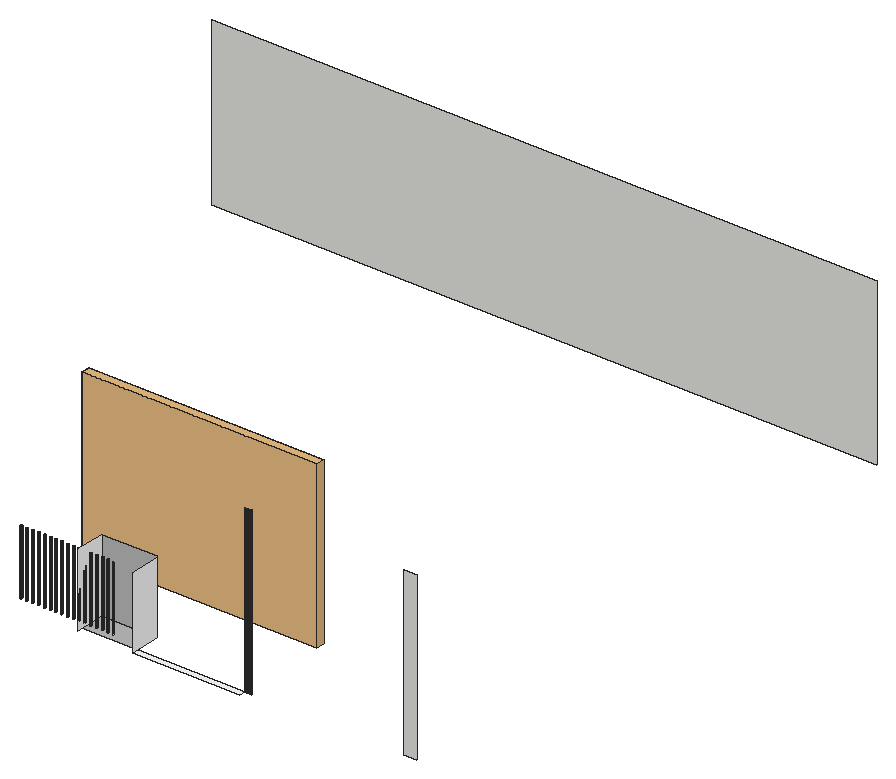
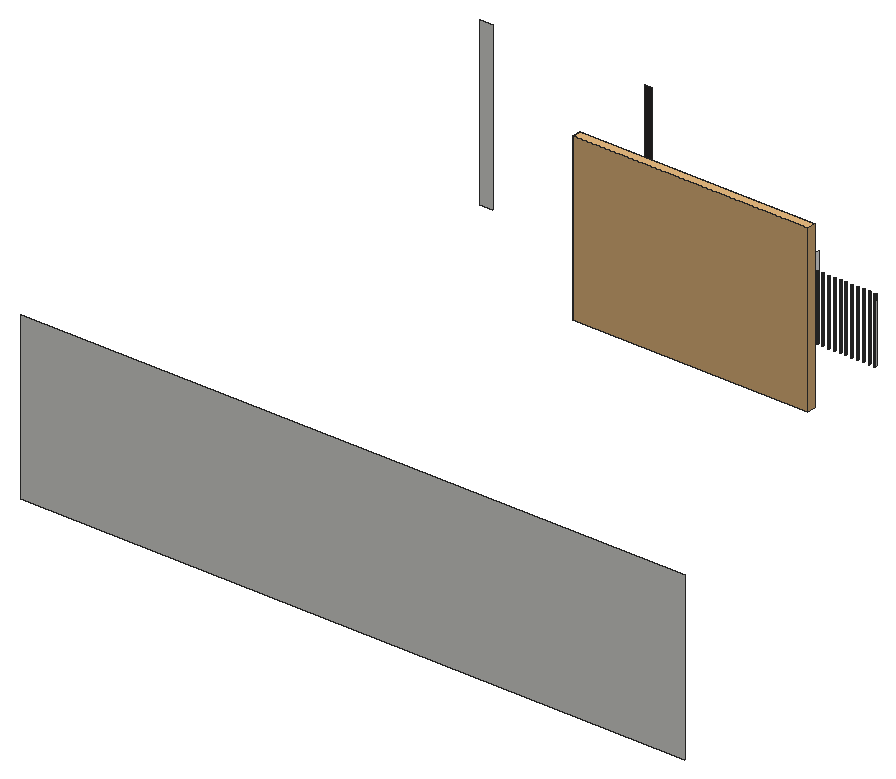
# SketchUp Ruby script. Lengths in inches.
U = 1.inch
M = Sketchup.active_model
def pt(a) = Geom::Point3d.new(a.map { |v| v * U })
def face(e, loops, mat)
  f = e.add_face(loops[0].map { |a| pt(a) })
  loops[1..].each { |l| e.add_face(l.map { |a| pt(a) }).erase! }
  f.material = f.back_material = mat if mat
  f
end
# faces: each face lists its corners as indices into pts; further lists are holes
def faces(e, pts, list, mat = nil) = list.each { |f| face(e, (f[0].is_a?(Array) ? f : [f]).map { |l| l.map { |i| pts[i] } }, mat) }
# xy, xz, yz: faces in a plane at the given z, y or x. An outline is a flat list of corners, or four numbers for a rectangle; further outlines are holes
def ring(l) = l.size == 4 ? [[l[0], l[1]], [l[2], l[1]], [l[2], l[3]], [l[0], l[3]]] : l.each_slice(2).to_a
def flat(e, list, mat, &to3) = list.each { |f| face(e, (f[0].is_a?(Array) ? f : [f]).map { |l| ring(l).map { |u, v| to3.(u, v) } }, mat) }
def xy(e, z, list, mat = nil) = flat(e, list, mat) { |x, y| [x, y, z] }
def xz(e, y, list, mat = nil) = flat(e, list, mat) { |x, z| [x, y, z] }
def yz(e, x, list, mat = nil) = flat(e, list, mat) { |y, z| [x, y, z] }
def lines(e, pts, list) = list.each { |a, b| e.add_line(pt(pts[a]), pt(pts[b])) }
# prism: a flat outline (further loops are holes) pulled along v
def prism(e, loops, v, mat = nil)
  f = face(e, loops, mat); d = Geom::Vector3d.new(v.map { |x| x * U })
  f.pushpull(f.normal.samedirection?(d) ? d.length : -d.length)
end
def box(e, o, s, mat = nil) = prism(e, [[o, [o[0] + s[0], o[1], o[2]], [o[0] + s[0], o[1] + s[1], o[2]], [o[0], o[1] + s[1], o[2]]]], [0, 0, s[2]], mat)
def at(x, y, z, deg = 0) = Geom::Transformation.translation(pt([x, y, z])) * Geom::Transformation.rotation(ORIGIN, Z_AXIS, deg.degrees)
def axes(o, x, y, z) = Geom::Transformation.new([*x, 0, *y, 0, *z, 0, *pt(o).to_a, 1])
def part(name) = M.definitions.add(name)
# library, detail: a bought-in or finely detailed component or shape, given as its bounding box
def library(name, o, s) = part(name).tap { |d| box(d.entities, o, s) }
def detail(e, o, s) = box(e.add_group.entities, o, s)
def put(e, d, t, mat = nil) = e.add_instance(d, t).tap { |i| i.material = mat if mat }
def group(e, t, mat = nil) = e.add_group.tap { |g| g.transformation = t; g.material = mat if mat }.entities
root = M.entities
M.materials.add("Generic\#2").color = [186, 186, 186]
M.materials.add("Generic\#4").color = [48, 45, 45]
M.materials.add("[Color M00]").color = [255, 255, 255]
c1 = library("Group\#9",[0,0,0],[238.3125,8.75,168])
xy(root,614.8125,[[294.98,132.01,294.77,132.04,294.58,132.125,294.41,132.25,294.28,132.42,294.2,132.62,294.17,132.83,294.2,133.04,294.28,133.23,294.41,133.4,294.58,133.53,294.77,133.61,294.98,133.64,295.19,133.61,295.39,133.53,295.56,133.4,295.6875,133.23,295.77,133.04,295.8,132.83,295.77,132.62,295.6875,132.42,295.56,132.25,295.39,132.125,295.19,132.04]])
xy(root,614.8125,[[363.4375,124.5,419.5625,149.5]],"Generic\#2")
xy(root,614.8125,[[419.5625,118.5625,528.75,124.5]],"[Color M00]")
xz(root,124.5,[[690.4375,614.8125,703.6875,782.8125]])
xz(root,124.5,[[528.75,614.8125,535.75,782.8125]],"Generic\#4")
xz(root,149.5,[[363.4375,614.8125,419.5625,689.33]],"Generic\#2")
xz(root,724.5,[[15.3125,614.8125,690.4375,782.8125]])
yz(root,363.4375,[[118.5625,614.8125,149.5,689.33]],"[Color M00]")
yz(root,419.5625,[[118.5625,614.8125,149.5,687.77]],"[Color M00]")
p = [[294.58,132.125,614.8125],[294.77,132.04,614.8125],[294.77,132.04,680.58],[294.58,132.125,680.58],[294.98,132.01,614.8125],[294.98,132.01,680.58],
  [295.19,132.04,614.8125],[295.19,132.04,680.58],[295.39,132.125,614.8125],[295.39,132.125,680.58],[300.58,132.125,614.8125],[300.77,132.04,614.8125],
  [300.77,132.04,680.58],[300.58,132.125,680.58],[300.98,132.01,614.8125],[300.98,132.01,680.58],[301.19,132.04,614.8125],[301.19,132.04,680.58],
  [301.39,132.125,614.8125],[301.39,132.125,680.58],[306.51,132.125,614.8125],[306.71,132.04,614.8125],[306.71,132.04,680.58],[306.51,132.125,680.58],
  [306.92,132.01,614.8125],[306.92,132.01,680.58],[307.13,132.04,614.8125],[307.13,132.04,680.58],[307.33,132.125,614.8125],[307.33,132.125,680.58],
  [312.39,132.125,614.8125],[312.58,132.04,614.8125],[312.58,132.04,680.58],[312.39,132.125,680.58],[312.8,132.01,614.8125],[312.8,132.01,680.58],
  [313.01,132.04,614.8125],[313.01,132.04,680.58],[313.2,132.125,614.8125],[313.2,132.125,680.58],[318.33,132.125,614.8125],[318.52,132.04,614.8125],
  [318.52,132.04,680.58],[318.33,132.125,680.58],[318.73,132.01,614.8125],[318.73,132.01,680.58],[318.94,132.04,614.8125],[318.94,132.04,680.58],
  [319.14,132.125,614.8125],[319.14,132.125,680.58],[324.58,132.125,614.8125],[324.77,132.04,614.8125],[324.77,132.04,680.58],[324.58,132.125,680.58],
  [324.98,132.01,614.8125],[324.98,132.01,680.58],[325.19,132.04,614.8125],[325.19,132.04,680.58],[325.39,132.125,614.8125],[325.39,132.125,680.58],
  [330.08,132.125,614.8125],[330.27,132.04,614.8125],[330.27,132.04,680.58],[330.08,132.125,680.58],[330.48,132.01,614.8125],[330.48,132.01,680.58],
  [330.69,132.04,614.8125],[330.69,132.04,680.58],[330.89,132.125,614.8125],[330.89,132.125,680.58],[336.14,132.07,614.8125],[336.36,132.04,614.8125],
  [336.36,132.04,680.58],[336.14,132.07,680.58],[336.57,132.07,614.8125],[336.57,132.07,680.58],[342.02,132.07,614.8125],[342.23,132.04,614.8125],
  [342.23,132.04,680.58],[342.02,132.07,680.58],[342.44,132.07,614.8125],[342.44,132.07,680.58],[348.02,132.07,614.8125],[348.23,132.04,614.8125],
  [348.23,132.04,680.58],[348.02,132.07,680.58],[348.44,132.07,614.8125],[348.44,132.07,680.58],[353.58,132.07,614.8125],[353.79,132.04,614.8125],
  [353.79,132.04,680.58],[353.58,132.07,680.58],[354,132.07,614.8125],[354,132.07,680.58],[359.64,132.07,614.8125],[359.86,132.04,614.8125],
  [359.86,132.04,680.58],[359.64,132.07,680.58],[360.07,132.07,614.8125],[360.07,132.07,680.58],[365.46,132.07,614.8125],[365.67,132.04,614.8125],
  [365.67,132.04,680.58],[365.46,132.07,680.58],[365.88,132.07,614.8125],[365.88,132.07,680.58],[371.27,132.07,614.8125],[371.48,132.04,614.8125],
  [371.48,132.04,680.58],[371.27,132.07,680.58],[371.69,132.07,614.8125],[371.69,132.07,680.58],[377.21,132.07,614.8125],[377.42,132.04,614.8125],
  [377.42,132.04,680.58],[377.21,132.07,680.58],[377.63,132.07,614.8125],[377.63,132.07,680.58],[383.02,132.07,614.8125],[383.23,132.04,614.8125],
  [383.23,132.04,680.58],[383.02,132.07,680.58],[383.44,132.07,614.8125],[383.44,132.07,680.58],[388.96,132.07,614.8125],[389.17,132.04,614.8125],
  [389.17,132.04,680.58],[388.96,132.07,680.58],[294.41,132.25,614.8125],[294.41,132.25,680.58],[295.56,132.25,614.8125],[295.56,132.25,680.58],
  [300.41,132.25,614.8125],[300.41,132.25,680.58],[301.56,132.25,614.8125],[301.56,132.25,680.58],[306.35,132.25,614.8125],[306.35,132.25,680.58],
  [307.49,132.25,614.8125],[307.49,132.25,680.58],[312.22,132.25,614.8125],[312.22,132.25,680.58],[313.37,132.25,614.8125],[313.37,132.25,680.58],
  [318.16,132.25,614.8125],[318.16,132.25,680.58],[319.31,132.25,614.8125],[319.31,132.25,680.58],[324.41,132.25,614.8125],[324.41,132.25,680.58],
  [325.56,132.25,614.8125],[325.56,132.25,680.58],[329.91,132.25,614.8125],[329.91,132.25,680.58],[331.06,132.25,614.8125],[331.06,132.25,680.58],
  [335.95,132.15,614.8125],[335.95,132.15,680.58],[336.76,132.15,614.8125],[336.76,132.15,680.58],[341.82,132.15,614.8125],[341.82,132.15,680.58],
  [342.64,132.15,614.8125],[342.64,132.15,680.58],[347.82,132.15,614.8125],[347.82,132.15,680.58],[348.64,132.15,614.8125],[348.64,132.15,680.58],
  [353.39,132.15,614.8125],[353.39,132.15,680.58],[354.2,132.15,614.8125],[354.2,132.15,680.58],[359.45,132.15,614.8125],[359.45,132.15,680.58],
  [360.26,132.15,614.8125],[360.26,132.15,680.58],[365.26,132.15,614.8125],[365.26,132.15,680.58],[366.07,132.15,614.8125],[366.07,132.15,680.58],
  [371.07,132.15,614.8125],[371.07,132.15,680.58],[371.89,132.15,614.8125],[371.89,132.15,680.58],[377.01,132.15,614.8125],[377.01,132.15,680.58],
  [377.82,132.15,614.8125],[377.82,132.15,680.58],[382.82,132.15,614.8125],[382.82,132.15,680.58],[383.64,132.15,614.8125],[383.64,132.15,680.58],
  [388.76,132.15,614.8125],[388.76,132.15,680.58],[335.78,132.28,614.8125],[335.78,132.28,680.58],[336.93,132.28,614.8125],[336.93,132.28,680.58],
  [341.66,132.28,614.8125],[341.66,132.28,680.58],[342.8,132.28,614.8125],[342.8,132.28,680.58],[347.66,132.28,614.8125],[347.66,132.28,680.58],
  [348.8,132.28,614.8125],[348.8,132.28,680.58],[353.22,132.28,614.8125],[353.22,132.28,680.58],[354.37,132.28,614.8125],[354.37,132.28,680.58],
  [359.28,132.28,614.8125],[359.28,132.28,680.58],[360.43,132.28,614.8125],[360.43,132.28,680.58],[365.09,132.28,614.8125],[365.09,132.28,680.58],
  [366.24,132.28,614.8125],[366.24,132.28,680.58],[370.91,132.28,614.8125],[370.91,132.28,680.58],[372.05,132.28,614.8125],[372.05,132.28,680.58],
  [376.84,132.28,614.8125],[376.84,132.28,680.58],[377.99,132.28,614.8125],[377.99,132.28,680.58],[382.66,132.28,614.8125],[382.66,132.28,680.58],
  [383.8,132.28,614.8125],[383.8,132.28,680.58],[388.59,132.28,614.8125],[388.59,132.28,680.58],[294.28,132.42,614.8125],[294.28,132.42,680.58],
  [295.6875,132.42,614.8125],[295.6875,132.42,680.58],[300.28,132.42,614.8125],[300.28,132.42,680.58],[301.6875,132.42,614.8125],[301.6875,132.42,680.58],
  [306.22,132.42,614.8125],[306.22,132.42,680.58],[307.625,132.42,614.8125],[307.625,132.42,680.58],[312.09,132.42,614.8125],[312.09,132.42,680.58],
  [313.5,132.42,614.8125],[313.5,132.42,680.58],[318.03,132.42,614.8125],[318.03,132.42,680.58],[319.4375,132.42,614.8125],[319.4375,132.42,680.58],
  [324.28,132.42,614.8125],[324.28,132.42,680.58],[325.6875,132.42,614.8125],[325.6875,132.42,680.58],[329.78,132.42,614.8125],[329.78,132.42,680.58],
  [331.1875,132.42,614.8125],[331.1875,132.42,680.58],[335.65,132.45,614.8125],[335.65,132.45,680.58],[337.06,132.45,614.8125],[337.06,132.45,680.58],
  [341.53,132.45,614.8125],[341.53,132.45,680.58],[342.93,132.45,614.8125],[342.93,132.45,680.58],[347.53,132.45,614.8125],[347.53,132.45,680.58],
  [348.93,132.45,614.8125],[348.93,132.45,680.58],[353.09,132.45,614.8125],[353.09,132.45,680.58],[354.5,132.45,614.8125],[354.5,132.45,680.58],
  [359.15,132.45,614.8125],[359.15,132.45,680.58],[360.56,132.45,614.8125],[360.56,132.45,680.58],[364.96,132.45,614.8125],[364.96,132.45,680.58],
  [366.37,132.45,614.8125],[366.37,132.45,680.58],[370.78,132.45,614.8125],[370.78,132.45,680.58],[372.18,132.45,614.8125],[372.18,132.45,680.58],
  [376.71,132.45,614.8125],[376.71,132.45,680.58],[378.12,132.45,614.8125],[378.12,132.45,680.58],[382.53,132.45,614.8125],[382.53,132.45,680.58],
  [383.93,132.45,614.8125],[383.93,132.45,680.58],[388.46,132.45,614.8125],[388.46,132.45,680.58],[294.2,132.62,614.8125],[294.2,132.62,680.58],
  [295.77,132.62,614.8125],[295.77,132.62,680.58],[300.2,132.62,614.8125],[300.2,132.62,680.58],[301.77,132.62,614.8125],[301.77,132.62,680.58],
  [306.14,132.62,614.8125],[306.14,132.62,680.58],[307.7,132.62,614.8125],[307.7,132.62,680.58],[312.01,132.62,614.8125],[312.01,132.62,680.58],
  [313.58,132.62,614.8125],[313.58,132.62,680.58],[317.95,132.62,614.8125],[317.95,132.62,680.58],[319.52,132.62,614.8125],[319.52,132.62,680.58],
  [324.2,132.62,614.8125],[324.2,132.62,680.58],[325.77,132.62,614.8125],[325.77,132.62,680.58],[329.7,132.62,614.8125],[329.7,132.62,680.58],
  [331.27,132.62,614.8125],[331.27,132.62,680.58],[335.57,132.64,614.8125],[335.57,132.64,680.58],[337.14,132.64,614.8125],[337.14,132.64,680.58],
  [341.45,132.64,614.8125],[341.45,132.64,680.58],[343.02,132.64,614.8125],[343.02,132.64,680.58],[347.45,132.64,614.8125],[347.45,132.64,680.58],
  [349.02,132.64,614.8125],[349.02,132.64,680.58],[353.01,132.64,614.8125],[353.01,132.64,680.58],[354.58,132.64,614.8125],[354.58,132.64,680.58],
  [359.07,132.64,614.8125],[359.07,132.64,680.58],[360.64,132.64,614.8125],[360.64,132.64,680.58],[364.88,132.64,614.8125],[364.88,132.64,680.58],
  [366.45,132.64,614.8125],[366.45,132.64,680.58],[370.7,132.64,614.8125],[370.7,132.64,680.58],[372.27,132.64,614.8125],[372.27,132.64,680.58],
  [376.63,132.64,614.8125],[376.63,132.64,680.58],[378.2,132.64,614.8125],[378.2,132.64,680.58],[382.45,132.64,614.8125],[382.45,132.64,680.58],
  [384.02,132.64,614.8125],[384.02,132.64,680.58],[388.38,132.64,614.8125],[388.38,132.64,680.58],[294.17,132.83,614.8125],[294.17,132.83,680.58],
  [295.8,132.83,614.8125],[295.8,132.83,680.58],[300.17,132.83,614.8125],[300.17,132.83,680.58],[301.8,132.83,614.8125],[301.8,132.83,680.58],
  [306.11,132.83,614.8125],[306.11,132.83,680.58],[307.73,132.83,614.8125],[307.73,132.83,680.58],[311.98,132.83,614.8125],[311.98,132.83,680.58],
  [313.61,132.83,614.8125],[313.61,132.83,680.58],[317.92,132.83,614.8125],[317.92,132.83,680.58],[319.55,132.83,614.8125],[319.55,132.83,680.58],
  [324.17,132.83,614.8125],[324.17,132.83,680.58],[325.8,132.83,614.8125],[325.8,132.83,680.58],[329.67,132.83,614.8125],[329.67,132.83,680.58],
  [331.3,132.83,614.8125],[331.3,132.83,680.58],[335.54,132.85,614.8125],[335.54,132.85,680.58],[337.17,132.85,614.8125],[337.17,132.85,680.58],
  [341.42,132.85,614.8125],[341.42,132.85,680.58],[343.04,132.85,614.8125],[343.04,132.85,680.58],[347.42,132.85,614.8125],[347.42,132.85,680.58],
  [349.04,132.85,614.8125],[349.04,132.85,680.58],[352.98,132.85,614.8125],[352.98,132.85,680.58],[354.61,132.85,614.8125],[354.61,132.85,680.58],
  [359.04,132.85,614.8125],[359.04,132.85,680.58],[360.67,132.85,614.8125],[360.67,132.85,680.58],[364.86,132.85,614.8125],[364.86,132.85,680.58],
  [366.48,132.85,614.8125],[366.48,132.85,680.58],[370.67,132.85,614.8125],[370.67,132.85,680.58],[372.29,132.85,614.8125],[372.29,132.85,680.58],
  [376.61,132.85,614.8125],[376.61,132.85,680.58],[378.23,132.85,614.8125],[378.23,132.85,680.58],[382.42,132.85,614.8125],[382.42,132.85,680.58],
  [384.04,132.85,614.8125],[384.04,132.85,680.58],[294.2,133.04,614.8125],[294.2,133.04,680.58],[295.77,133.04,614.8125],[295.77,133.04,680.58],
  [300.2,133.04,614.8125],[300.2,133.04,680.58],[301.77,133.04,614.8125],[301.77,133.04,680.58],[306.14,133.04,614.8125],[306.14,133.04,680.58],
  [307.7,133.04,614.8125],[307.7,133.04,680.58],[312.01,133.04,614.8125],[312.01,133.04,680.58],[313.58,133.04,614.8125],[313.58,133.04,680.58],
  [317.95,133.04,614.8125],[317.95,133.04,680.58],[319.52,133.04,614.8125],[319.52,133.04,680.58],[324.2,133.04,614.8125],[324.2,133.04,680.58],
  [325.77,133.04,614.8125],[325.77,133.04,680.58],[329.7,133.04,614.8125],[329.7,133.04,680.58],[331.27,133.04,614.8125],[331.27,133.04,680.58],
  [335.57,133.06,614.8125],[335.57,133.06,680.58],[337.14,133.06,614.8125],[337.14,133.06,680.58],[341.45,133.06,614.8125],[341.45,133.06,680.58],
  [343.02,133.06,614.8125],[343.02,133.06,680.58],[347.45,133.06,614.8125],[347.45,133.06,680.58],[349.02,133.06,614.8125],[349.02,133.06,680.58],
  [353.01,133.06,614.8125],[353.01,133.06,680.58],[354.58,133.06,614.8125],[354.58,133.06,680.58],[359.07,133.06,614.8125],[359.07,133.06,680.58],
  [360.64,133.06,614.8125],[360.64,133.06,680.58],[364.88,133.06,614.8125],[364.88,133.06,680.58],[366.45,133.06,614.8125],[366.45,133.06,680.58],
  [370.7,133.06,614.8125],[370.7,133.06,680.58],[372.27,133.06,614.8125],[372.27,133.06,680.58],[376.63,133.06,614.8125],[376.63,133.06,680.58],
  [378.2,133.06,614.8125],[378.2,133.06,680.58],[382.45,133.06,614.8125],[382.45,133.06,680.58],[384.02,133.06,614.8125],[384.02,133.06,680.58],
  [294.28,133.23,614.8125],[294.28,133.23,680.58],[295.6875,133.23,614.8125],[295.6875,133.23,680.58],[300.28,133.23,614.8125],[300.28,133.23,680.58],
  [301.6875,133.23,614.8125],[301.6875,133.23,680.58],[306.22,133.23,614.8125],[306.22,133.23,680.58],[307.625,133.23,614.8125],[307.625,133.23,680.58],
  [312.09,133.23,614.8125],[312.09,133.23,680.58],[313.5,133.23,614.8125],[313.5,133.23,680.58],[318.03,133.23,614.8125],[318.03,133.23,680.58],
  [319.4375,133.23,614.8125],[319.4375,133.23,680.58],[324.28,133.23,614.8125],[324.28,133.23,680.58],[325.6875,133.23,614.8125],[325.6875,133.23,680.58],
  [329.78,133.23,614.8125],[329.78,133.23,680.58],[331.1875,133.23,614.8125],[331.1875,133.23,680.58],[335.65,133.26,614.8125],[335.65,133.26,680.58],
  [337.06,133.26,614.8125],[337.06,133.26,680.58],[341.53,133.26,614.8125],[341.53,133.26,680.58],[342.93,133.26,614.8125],[342.93,133.26,680.58],
  [347.53,133.26,614.8125],[347.53,133.26,680.58],[348.93,133.26,614.8125],[348.93,133.26,680.58],[353.09,133.26,614.8125],[353.09,133.26,680.58],
  [354.5,133.26,614.8125],[354.5,133.26,680.58],[359.15,133.26,614.8125],[359.15,133.26,680.58],[360.56,133.26,614.8125],[360.56,133.26,680.58],
  [364.96,133.26,614.8125],[364.96,133.26,680.58],[366.37,133.26,614.8125],[366.37,133.26,680.58],[370.78,133.26,614.8125],[370.78,133.26,680.58],
  [372.18,133.26,614.8125],[372.18,133.26,680.58],[376.71,133.26,614.8125],[376.71,133.26,680.58],[378.12,133.26,614.8125],[378.12,133.26,680.58],
  [382.53,133.26,614.8125],[382.53,133.26,680.58],[383.93,133.26,614.8125],[383.93,133.26,680.58],[294.41,133.4,614.8125],[294.41,133.4,680.58],
  [295.56,133.4,614.8125],[295.56,133.4,680.58],[300.41,133.4,614.8125],[300.41,133.4,680.58],[301.56,133.4,614.8125],[301.56,133.4,680.58],
  [306.35,133.4,614.8125],[306.35,133.4,680.58],[307.49,133.4,614.8125],[307.49,133.4,680.58],[312.22,133.4,614.8125],[312.22,133.4,680.58],
  [313.37,133.4,614.8125],[313.37,133.4,680.58],[318.16,133.4,614.8125],[318.16,133.4,680.58],[319.31,133.4,614.8125],[319.31,133.4,680.58],
  [324.41,133.4,614.8125],[324.41,133.4,680.58],[325.56,133.4,614.8125],[325.56,133.4,680.58],[329.91,133.4,614.8125],[329.91,133.4,680.58],
  [331.06,133.4,614.8125],[331.06,133.4,680.58],[335.78,133.43,614.8125],[335.78,133.43,680.58],[336.93,133.43,614.8125],[336.93,133.43,680.58],
  [341.66,133.43,614.8125],[341.66,133.43,680.58],[342.8,133.43,614.8125],[342.8,133.43,680.58],[347.66,133.43,614.8125],[347.66,133.43,680.58],
  [348.8,133.43,614.8125],[348.8,133.43,680.58],[353.22,133.43,614.8125],[353.22,133.43,680.58],[354.37,133.43,614.8125],[354.37,133.43,680.58],
  [359.28,133.43,614.8125],[359.28,133.43,680.58],[360.43,133.43,614.8125],[360.43,133.43,680.58],[365.09,133.43,614.8125],[365.09,133.43,680.58],
  [366.24,133.43,614.8125],[366.24,133.43,680.58],[370.91,133.43,614.8125],[370.91,133.43,680.58],[372.05,133.43,614.8125],[372.05,133.43,680.58],
  [376.84,133.43,614.8125],[376.84,133.43,680.58],[377.99,133.43,614.8125],[377.99,133.43,680.58],[382.66,133.43,614.8125],[382.66,133.43,680.58],
  [383.8,133.43,614.8125],[383.8,133.43,680.58],[294.58,133.53,614.8125],[294.58,133.53,680.58],[295.39,133.53,614.8125],[295.39,133.53,680.58],
  [300.58,133.53,614.8125],[300.58,133.53,680.58],[301.39,133.53,614.8125],[301.39,133.53,680.58],[306.51,133.53,614.8125],[306.51,133.53,680.58],
  [307.33,133.53,614.8125],[307.33,133.53,680.58],[312.39,133.53,614.8125],[312.39,133.53,680.58],[313.2,133.53,614.8125],[313.2,133.53,680.58],
  [318.33,133.53,614.8125],[318.33,133.53,680.58],[319.14,133.53,614.8125],[319.14,133.53,680.58],[324.58,133.53,614.8125],[324.58,133.53,680.58],
  [325.39,133.53,614.8125],[325.39,133.53,680.58],[330.08,133.53,614.8125],[330.08,133.53,680.58],[330.89,133.53,614.8125],[330.89,133.53,680.58],
  [335.95,133.56,614.8125],[335.95,133.56,680.58],[336.76,133.56,614.8125],[336.76,133.56,680.58],[341.82,133.56,614.8125],[341.82,133.56,680.58],
  [342.64,133.56,614.8125],[342.64,133.56,680.58],[347.82,133.56,614.8125],[347.82,133.56,680.58],[348.64,133.56,614.8125],[348.64,133.56,680.58],
  [353.39,133.56,614.8125],[353.39,133.56,680.58],[354.2,133.56,614.8125],[354.2,133.56,680.58],[359.45,133.56,614.8125],[359.45,133.56,680.58],
  [360.26,133.56,614.8125],[360.26,133.56,680.58],[365.26,133.56,614.8125],[365.26,133.56,680.58],[366.07,133.56,614.8125],[366.07,133.56,680.58],
  [371.07,133.56,614.8125],[371.07,133.56,680.58],[371.89,133.56,614.8125],[371.89,133.56,680.58],[377.01,133.56,614.8125],[377.01,133.56,680.58],
  [377.82,133.56,614.8125],[377.82,133.56,680.58],[382.82,133.56,614.8125],[382.82,133.56,680.58],[383.64,133.56,614.8125],[383.64,133.56,680.58],
  [294.77,133.61,614.8125],[294.77,133.61,680.58],[295.19,133.61,614.8125],[295.19,133.61,680.58],[300.77,133.61,614.8125],[300.77,133.61,680.58],
  [301.19,133.61,614.8125],[301.19,133.61,680.58],[306.71,133.61,614.8125],[306.71,133.61,680.58],[307.13,133.61,614.8125],[307.13,133.61,680.58],
  [312.58,133.61,614.8125],[312.58,133.61,680.58],[313.01,133.61,614.8125],[313.01,133.61,680.58],[318.52,133.61,614.8125],[318.52,133.61,680.58],
  [318.94,133.61,614.8125],[318.94,133.61,680.58],[324.77,133.61,614.8125],[324.77,133.61,680.58],[325.19,133.61,614.8125],[325.19,133.61,680.58],
  [330.27,133.61,614.8125],[330.27,133.61,680.58],[330.69,133.61,614.8125],[330.69,133.61,680.58],[294.98,133.64,614.8125],[294.98,133.64,680.58],
  [300.98,133.64,614.8125],[300.98,133.64,680.58],[306.92,133.64,614.8125],[306.92,133.64,680.58],[312.8,133.64,614.8125],[312.8,133.64,680.58],
  [318.73,133.64,614.8125],[318.73,133.64,680.58],[324.98,133.64,614.8125],[324.98,133.64,680.58],[330.48,133.64,614.8125],[330.48,133.64,680.58],
  [336.14,133.64,614.8125],[336.14,133.64,680.58],[336.36,133.67,614.8125],[336.36,133.67,680.58],[336.57,133.64,614.8125],[336.57,133.64,680.58],
  [342.02,133.64,614.8125],[342.02,133.64,680.58],[342.23,133.67,614.8125],[342.23,133.67,680.58],[342.44,133.64,614.8125],[342.44,133.64,680.58],
  [348.02,133.64,614.8125],[348.02,133.64,680.58],[348.23,133.67,614.8125],[348.23,133.67,680.58],[348.44,133.64,614.8125],[348.44,133.64,680.58],
  [353.58,133.64,614.8125],[353.58,133.64,680.58],[353.79,133.67,614.8125],[353.79,133.67,680.58],[354,133.64,614.8125],[354,133.64,680.58],
  [359.64,133.64,614.8125],[359.64,133.64,680.58],[359.86,133.67,614.8125],[359.86,133.67,680.58],[360.07,133.64,614.8125],[360.07,133.64,680.58],
  [365.46,133.64,614.8125],[365.46,133.64,680.58],[365.67,133.67,614.8125],[365.67,133.67,680.58],[365.88,133.64,614.8125],[365.88,133.64,680.58],
  [371.27,133.64,614.8125],[371.27,133.64,680.58],[371.48,133.67,614.8125],[371.48,133.67,680.58],[371.69,133.64,614.8125],[371.69,133.64,680.58],
  [377.21,133.64,614.8125],[377.21,133.64,680.58],[377.42,133.67,614.8125],[377.42,133.67,680.58],[377.63,133.64,614.8125],[377.63,133.64,680.58],
  [383.02,133.64,614.8125],[383.02,133.64,680.58],[383.23,133.67,614.8125],[383.23,133.67,680.58],[383.44,133.64,614.8125],[383.44,133.64,680.58]]
faces(root,p,[[0,1,2,3],[1,4,5,2],[4,6,7,5],[6,8,9,7],[10,11,12,13],[11,14,15,12],[14,16,17,15],[16,18,19,17],
  [20,21,22,23],[21,24,25,22],[24,26,27,25],[26,28,29,27],[30,31,32,33],[31,34,35,32],[34,36,37,35],[36,38,39,37],
  [40,41,42,43],[41,44,45,42],[44,46,47,45],[46,48,49,47],[50,51,52,53],[51,54,55,52],[54,56,57,55],[56,58,59,57],
  [60,61,62,63],[61,64,65,62],[64,66,67,65],[66,68,69,67],[70,71,72,73],[71,74,75,72],[76,77,78,79],[77,80,81,78],
  [82,83,84,85],[83,86,87,84],[88,89,90,91],[89,92,93,90],[94,95,96,97],[95,98,99,96],[100,101,102,103],[101,104,105,102],
  [106,107,108,109],[107,110,111,108],[112,113,114,115],[113,116,117,114],[118,119,120,121],[119,122,123,120],[124,125,126,127],[128,0,3,129],
  [8,130,131,9],[132,10,13,133],[18,134,135,19],[136,20,23,137],[28,138,139,29],[140,30,33,141],[38,142,143,39],[144,40,43,145],
  [48,146,147,49],[148,50,53,149],[58,150,151,59],[152,60,63,153],[68,154,155,69],[156,70,73,157],[74,158,159,75],[160,76,79,161],
  [80,162,163,81],[164,82,85,165],[86,166,167,87],[168,88,91,169],[92,170,171,93],[172,94,97,173],[98,174,175,99],[176,100,103,177],
  [104,178,179,105],[180,106,109,181],[110,182,183,111],[184,112,115,185],[116,186,187,117],[188,118,121,189],[122,190,191,123],[192,124,127,193],
  [194,156,157,195],[158,196,197,159],[198,160,161,199],[162,200,201,163],[202,164,165,203],[166,204,205,167],[206,168,169,207],[170,208,209,171],
  [210,172,173,211],[174,212,213,175],[214,176,177,215],[178,216,217,179],[218,180,181,219],[182,220,221,183],[222,184,185,223],[186,224,225,187],
  [226,188,189,227],[190,228,229,191],[230,192,193,231],[232,128,129,233],[130,234,235,131],[236,132,133,237],[134,238,239,135],[240,136,137,241],
  [138,242,243,139],[244,140,141,245],[142,246,247,143],[248,144,145,249],[146,250,251,147],[252,148,149,253],[150,254,255,151],[256,152,153,257],
  [154,258,259,155],[260,194,195,261],[196,262,263,197],[264,198,199,265],[200,266,267,201],[268,202,203,269],[204,270,271,205],[272,206,207,273],
  [208,274,275,209],[276,210,211,277],[212,278,279,213],[280,214,215,281],[216,282,283,217],[284,218,219,285],[220,286,287,221],[288,222,223,289],
  [224,290,291,225],[292,226,227,293],[228,294,295,229],[296,230,231,297],[298,232,233,299],[234,300,301,235],[302,236,237,303],[238,304,305,239],
  [306,240,241,307],[242,308,309,243],[310,244,245,311],[246,312,313,247],[314,248,249,315],[250,316,317,251],[318,252,253,319],[254,320,321,255],
  [322,256,257,323],[258,324,325,259],[326,260,261,327],[262,328,329,263],[330,264,265,331],[266,332,333,267],[334,268,269,335],[270,336,337,271],
  [338,272,273,339],[274,340,341,275],[342,276,277,343],[278,344,345,279],[346,280,281,347],[282,348,349,283],[350,284,285,351],[286,352,353,287],
  [354,288,289,355],[290,356,357,291],[358,292,293,359],[294,360,361,295],[362,296,297,363],[364,298,299,365],[300,366,367,301],[368,302,303,369],
  [304,370,371,305],[372,306,307,373],[308,374,375,309],[376,310,311,377],[312,378,379,313],[380,314,315,381],[316,382,383,317],[384,318,319,385],
  [320,386,387,321],[388,322,323,389],[324,390,391,325],[392,326,327,393],[328,394,395,329],[396,330,331,397],[332,398,399,333],[400,334,335,401],
  [336,402,403,337],[404,338,339,405],[340,406,407,341],[408,342,343,409],[344,410,411,345],[412,346,347,413],[348,414,415,349],[416,350,351,417],
  [352,418,419,353],[420,354,355,421],[356,422,423,357],[424,358,359,425],[360,426,427,361],[428,364,365,429],[366,430,431,367],[432,368,369,433],
  [370,434,435,371],[436,372,373,437],[374,438,439,375],[440,376,377,441],[378,442,443,379],[444,380,381,445],[382,446,447,383],[448,384,385,449],
  [386,450,451,387],[452,388,389,453],[390,454,455,391],[456,392,393,457],[394,458,459,395],[460,396,397,461],[398,462,463,399],[464,400,401,465],
  [402,466,467,403],[468,404,405,469],[406,470,471,407],[472,408,409,473],[410,474,475,411],[476,412,413,477],[414,478,479,415],[480,416,417,481],
  [418,482,483,419],[484,420,421,485],[422,486,487,423],[488,424,425,489],[426,490,491,427],[492,428,429,493],[430,494,495,431],[496,432,433,497],
  [434,498,499,435],[500,436,437,501],[438,502,503,439],[504,440,441,505],[442,506,507,443],[508,444,445,509],[446,510,511,447],[512,448,449,513],
  [450,514,515,451],[516,452,453,517],[454,518,519,455],[520,456,457,521],[458,522,523,459],[524,460,461,525],[462,526,527,463],[528,464,465,529],
  [466,530,531,467],[532,468,469,533],[470,534,535,471],[536,472,473,537],[474,538,539,475],[540,476,477,541],[478,542,543,479],[544,480,481,545],
  [482,546,547,483],[548,484,485,549],[486,550,551,487],[552,488,489,553],[490,554,555,491],[556,492,493,557],[494,558,559,495],[560,496,497,561],
  [498,562,563,499],[564,500,501,565],[502,566,567,503],[568,504,505,569],[506,570,571,507],[572,508,509,573],[510,574,575,511],[576,512,513,577],
  [514,578,579,515],[580,516,517,581],[518,582,583,519],[584,520,521,585],[522,586,587,523],[588,524,525,589],[526,590,591,527],[592,528,529,593],
  [530,594,595,531],[596,532,533,597],[534,598,599,535],[600,536,537,601],[538,602,603,539],[604,540,541,605],[542,606,607,543],[608,544,545,609],
  [546,610,611,547],[612,548,549,613],[550,614,615,551],[616,552,553,617],[554,618,619,555],[620,556,557,621],[558,622,623,559],[624,560,561,625],
  [562,626,627,563],[628,564,565,629],[566,630,631,567],[632,568,569,633],[570,634,635,571],[636,572,573,637],[574,638,639,575],[640,576,577,641],
  [578,642,643,579],[644,580,581,645],[582,646,647,583],[648,584,585,649],[586,650,651,587],[652,588,589,653],[590,654,655,591],[656,592,593,657],
  [594,658,659,595],[660,596,597,661],[598,662,663,599],[664,600,601,665],[602,666,667,603],[668,604,605,669],[606,670,671,607],[672,608,609,673],
  [610,674,675,611],[676,612,613,677],[614,678,679,615],[680,616,617,681],[618,682,683,619],[684,620,621,685],[622,686,687,623],[688,624,625,689],
  [626,690,691,627],[692,628,629,693],[630,694,695,631],[696,632,633,697],[634,698,699,635],[700,636,637,701],[638,702,703,639],[704,640,641,705],
  [642,706,707,643],[708,644,645,709],[646,710,711,647],[712,684,685,713],[686,712,713,687],[714,688,689,715],[690,714,715,691],[716,692,693,717],
  [694,716,717,695],[718,696,697,719],[698,718,719,699],[720,700,701,721],[702,720,721,703],[722,704,705,723],[706,722,723,707],[724,708,709,725],
  [710,724,725,711],[726,648,649,727],[728,726,727,729],[730,728,729,731],[650,730,731,651],[732,652,653,733],[734,732,733,735],[736,734,735,737],
  [654,736,737,655],[738,656,657,739],[740,738,739,741],[742,740,741,743],[658,742,743,659],[744,660,661,745],[746,744,745,747],[748,746,747,749],
  [662,748,749,663],[750,664,665,751],[752,750,751,753],[754,752,753,755],[666,754,755,667],[756,668,669,757],[758,756,757,759],[760,758,759,761],
  [670,760,761,671],[762,672,673,763],[764,762,763,765],[766,764,765,767],[674,766,767,675],[768,676,677,769],[770,768,769,771],[772,770,771,773],
  [678,772,773,679],[774,680,681,775],[776,774,775,777],[778,776,777,779],[682,778,779,683]])
put(root,c1,at(290.4375,215.5625,614.8125))
